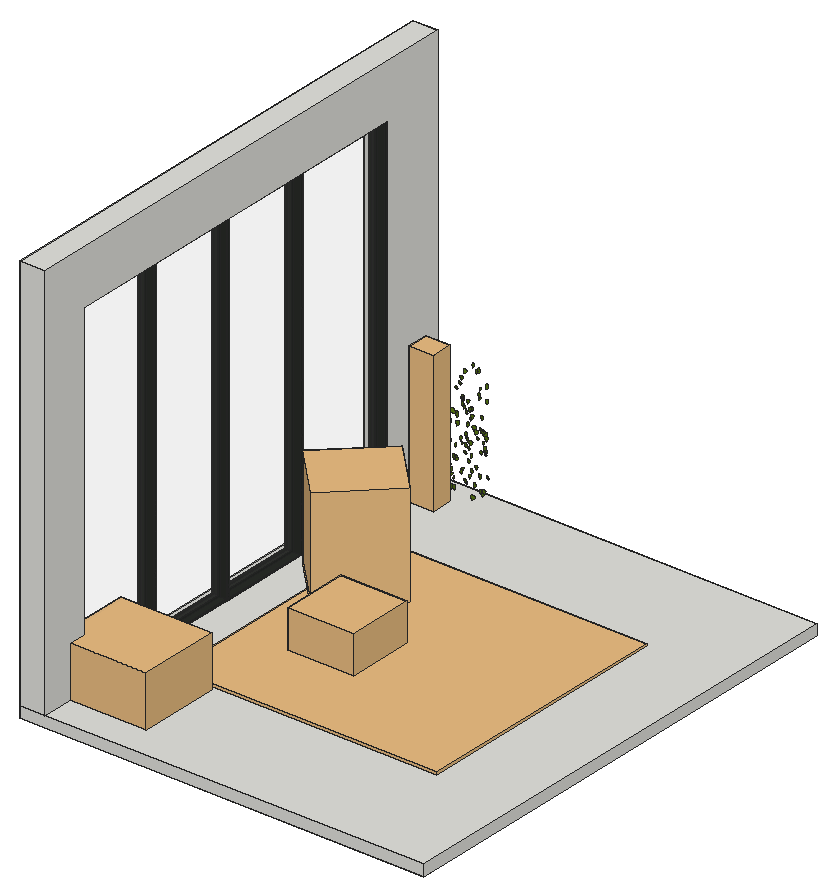
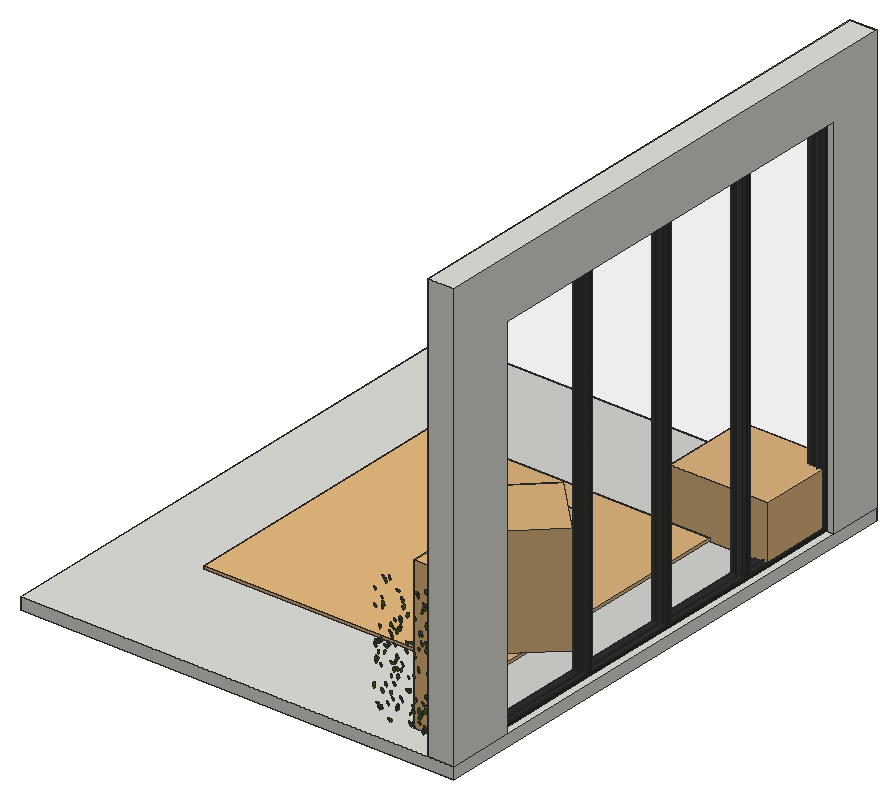
# SketchUp Ruby script. Lengths in inches.
U = 1.inch
M = Sketchup.active_model
def pt(a) = Geom::Point3d.new(a.map { |v| v * U })
def face(e, loops, mat)
  f = e.add_face(loops[0].map { |a| pt(a) })
  loops[1..].each { |l| e.add_face(l.map { |a| pt(a) }).erase! }
  f.material = f.back_material = mat if mat
  f
end
# faces: each face lists its corners as indices into pts; further lists are holes
def faces(e, pts, list, mat = nil) = list.each { |f| face(e, (f[0].is_a?(Array) ? f : [f]).map { |l| l.map { |i| pts[i] } }, mat) }
# xy, xz, yz: faces in a plane at the given z, y or x. An outline is a flat list of corners, or four numbers for a rectangle; further outlines are holes
def ring(l) = l.size == 4 ? [[l[0], l[1]], [l[2], l[1]], [l[2], l[3]], [l[0], l[3]]] : l.each_slice(2).to_a
def flat(e, list, mat, &to3) = list.each { |f| face(e, (f[0].is_a?(Array) ? f : [f]).map { |l| ring(l).map { |u, v| to3.(u, v) } }, mat) }
def xy(e, z, list, mat = nil) = flat(e, list, mat) { |x, y| [x, y, z] }
def xz(e, y, list, mat = nil) = flat(e, list, mat) { |x, z| [x, y, z] }
def yz(e, x, list, mat = nil) = flat(e, list, mat) { |y, z| [x, y, z] }
def lines(e, pts, list) = list.each { |a, b| e.add_line(pt(pts[a]), pt(pts[b])) }
# prism: a flat outline (further loops are holes) pulled along v
def prism(e, loops, v, mat = nil)
  f = face(e, loops, mat); d = Geom::Vector3d.new(v.map { |x| x * U })
  f.pushpull(f.normal.samedirection?(d) ? d.length : -d.length)
end
def box(e, o, s, mat = nil) = prism(e, [[o, [o[0] + s[0], o[1], o[2]], [o[0] + s[0], o[1] + s[1], o[2]], [o[0], o[1] + s[1], o[2]]]], [0, 0, s[2]], mat)
def at(x, y, z, deg = 0) = Geom::Transformation.translation(pt([x, y, z])) * Geom::Transformation.rotation(ORIGIN, Z_AXIS, deg.degrees)
def axes(o, x, y, z) = Geom::Transformation.new([*x, 0, *y, 0, *z, 0, *pt(o).to_a, 1])
def part(name) = M.definitions.add(name)
# library, detail: a bought-in or finely detailed component or shape, given as its bounding box
def library(name, o, s) = part(name).tap { |d| box(d.entities, o, s) }
def detail(e, o, s) = box(e.add_group.entities, o, s)
def put(e, d, t, mat = nil) = e.add_instance(d, t).tap { |i| i.material = mat if mat }
def group(e, t, mat = nil) = e.add_group.tap { |g| g.transformation = t; g.material = mat if mat }.entities
root = M.entities
M.materials.add("Glazing").color = [128, 128, 128]
M.materials["Glazing"].alpha = 0.05
M.materials.add("Powdercoating").color = [41, 44, 40]
M.materials.add("[Vegetation Blur 03]").color = [83, 114, 18]
M.materials.add("grey velvet texture").color = [200, 200, 193]
c1 = library("Potted plant",[-17.58,-15.45,-0.53],[33.42,30.09,19.21])
c2 = library("07",[-18.99,-18.99,0],[37.98,37.98,14.32])
c3 = part("Group\#15")
xy(c3.entities,0,[[0,-55.94,0.71,45.94]])
xy(c3.entities,0.2,[[0,-55.94,0.47,45.94],[0.47,45.94,0.71,46.42]])
xy(c3.entities,2.36,[[0.47,-55.94,0.71,46.42]])
xz(c3.entities,-55.94,[[0,0,0.71,0,0.71,2.36,0.47,2.36,0.47,0.2,0,0.2]])
xz(c3.entities,45.94,[[0,0,0.71,0.2]])
xz(c3.entities,46.42,[[0.47,0.2,0.71,2.36]])
yz(c3.entities,0,[[-55.94,0,45.94,0.2]])
yz(c3.entities,0.47,[[-55.94,0.2,46.42,2.36]])
yz(c3.entities,0.71,[[-55.94,0,45.94,0,45.94,0.2,46.42,0.2,46.42,2.36,-55.94,2.36]])
c4 = part("Group\#7")
xy(c4.entities,0,[[0,-59.09,0.71,45.94]])
xy(c4.entities,0.2,[[0,-59.09,0.47,45.94],[0.47,45.94,0.71,46.42]])
xy(c4.entities,2.36,[[0.47,-59.09,0.71,46.42]])
xz(c4.entities,-59.09,[[0,0,0.71,0,0.71,2.36,0.47,2.36,0.47,0.2,0,0.2]])
xz(c4.entities,45.94,[[0,0,0.71,0.2]])
xz(c4.entities,46.42,[[0.47,0.2,0.71,2.36]])
yz(c4.entities,0,[[-59.09,0,45.94,0.2]])
yz(c4.entities,0.47,[[-59.09,0.2,46.42,2.36]])
yz(c4.entities,0.71,[[-59.09,0,45.94,0,45.94,0.2,46.42,0.2,46.42,2.36,-59.09,2.36]])
c5 = part("Group\#16")
prism(c5.entities,[[[0.47,-56.18,0.2],[0,-56.18,0.2],[0,-56.18,0],[0.71,-56.18,0],[0.71,-56.18,2.36],[0.47,-56.18,2.36]]],[0,28.68,0])
c6 = part("Group\#10")
box(c6.entities,[-0.73,0,0],[27.99,0.55,102.05])
c7 = part("Group\#18")
xy(c7.entities,0,[[0.47,-56.18,0.47,-55.47,0,-55.47,0,-28.21,1.18,-28.21,1.18,-56.18]])
xy(c7.entities,0.2,[[0.71,-56.18,1.18,-28.21],[0,-55.47,0.47,-28.21],[0.47,-28.21,0.71,-27.74]])
xy(c7.entities,2.36,[[0.47,-56.18,0.71,-27.74]])
xz(c7.entities,-56.18,[[0.47,0,1.18,0,1.18,0.2,0.71,0.2,0.71,2.36,0.47,2.36]])
xz(c7.entities,-55.47,[[0,0,0.47,0.2]])
xz(c7.entities,-28.21,[[0,0,1.18,0.2]])
xz(c7.entities,-27.74,[[0.47,0.2,0.71,2.36]])
yz(c7.entities,0,[[-55.47,0,-28.21,0.2]])
yz(c7.entities,0.47,[[-56.18,0,-55.47,0.2],[-56.18,0.2,-27.74,2.36]])
yz(c7.entities,0.71,[[-56.18,0.2,-27.74,2.36]])
yz(c7.entities,1.18,[[-56.18,0,-28.21,0.2]])
c8 = part("Group\#34")
xy(c8.entities,0,[[-20.45,0,7.76,1.22]])
xy(c8.entities,0.06,[[-20.39,0.06,7.7,1.22]])
xy(c8.entities,0.47,[[-19.98,0,7.28,0.06]])
xy(c8.entities,101.89,[[-19.98,0,7.28,0.06]])
xy(c8.entities,102.3,[[-20.39,0.06,7.7,1.22]])
xy(c8.entities,102.36,[[-20.45,0,7.76,1.22]])
xz(c8.entities,0,[[[-20.45,0,7.76,102.36],[-19.98,0.47,7.28,101.89]]])
xz(c8.entities,0.06,[[[-20.39,0.06,7.7,102.3],[-19.98,0.47,7.28,101.89]]])
xz(c8.entities,1.22,[[[-20.45,0,7.76,102.36],[-20.39,0.06,7.7,102.3]]])
yz(c8.entities,-20.45,[[0,0,1.22,102.36]])
yz(c8.entities,-20.39,[[0.06,0.06,1.22,102.3]])
yz(c8.entities,-19.98,[[0,0.47,0.06,101.89]])
yz(c8.entities,7.28,[[0,0.47,0.06,101.89]])
yz(c8.entities,7.7,[[0.06,0.06,1.22,102.3]])
yz(c8.entities,7.76,[[0,0,1.22,102.36]])
c9 = part("Group\#6")
put(c9.entities,c3,axes([27.97,0,7.875],[1,0,0],[0,0,-1],[0,1,0]),"Powdercoating")
put(c9.entities,c4,axes([0.71,0,6.8],[-1,0,0],[0,0,-0.97687],[0,1,0]),"Powdercoating")
put(c9.entities,c5,axes([-27.5,0,-38.07],[0,0,-1],[-1,0,0],[0,1,0]),"Powdercoating")
put(c9.entities,c6,at(1.12,0.35,-38.39),"Glazing")
put(c9.entities,c7,axes([-27.5,0,63.35],[0,0,1],[-1,0,0],[0,1,0]),"Powdercoating")
put(c9.entities,c8,at(20.6875,1.0625,-38.54),"Powdercoating")
c10 = part("Sliding door panels")
put(c10.entities,c9,at(-1.18,4.5,38.86))
g1 = group(c10.entities,at(84.74,4.5,38.86))
put(g1,c3,axes([-27.97,0,7.875],[-1,0,0],[0,0,-1],[0,1,0]),"Powdercoating")
put(g1,c4,axes([-0.71,0,6.8],[1,0,0],[0,0,-0.97687],[0,1,0]),"Powdercoating")
put(g1,c5,axes([27.5,0,-38.07],[0,0,-1],[1,0,0],[0,1,0]),"Powdercoating")
put(g1,c6,axes([-1.12,0.35,-38.39],[-1,0,0],[0,1,0],[0,0,1]),"Glazing")
put(g1,c7,axes([27.5,0,63.35],[0,0,1],[1,0,0],[0,1,0]),"Powdercoating")
put(g1,c8,axes([-20.6875,1.0625,-38.54],[-1,0,0],[0,1,0],[0,0,1]),"Powdercoating")
g2 = group(c10.entities,at(56.0625,4.5,38.86))
put(g2,c3,axes([-27.97,0,7.875],[-1,0,0],[0,0,-1],[0,1,0]),"Powdercoating")
put(g2,c5,axes([27.5,0,-38.07],[0,0,-1],[1,0,0],[0,1,0]),"Powdercoating")
put(g2,c6,axes([-1.12,0.35,-38.39],[-1,0,0],[0,1,0],[0,0,1]),"Glazing")
put(g2,c7,axes([27.5,0,63.35],[0,0,1],[1,0,0],[0,1,0]),"Powdercoating")
put(g2,c8,axes([-20.6875,1.0625,-38.54],[-1,0,0],[0,1,0],[0,0,1]),"Powdercoating")
g3 = group(g2,at(-0.71,0,6.8),"Powdercoating")
xy(g3,-45.34,[[0.47,0.2,0.71,2.36]])
xy(g3,-44.88,[[0,0,0.71,0.2]])
xy(g3,57.73,[[0,0,0.71,0,0.71,2.36,0.47,2.36,0.47,0.2,0,0.2]])
xz(g3,0,[[0,-44.88,0.71,57.73]])
xz(g3,0.2,[[0.47,-45.34,0.71,-44.88],[0,-44.88,0.47,57.73]])
xz(g3,2.36,[[0.47,-45.34,0.71,57.73]])
yz(g3,0,[[0,-44.88,0.2,57.73]])
yz(g3,0.47,[[0.2,-45.34,2.36,57.73]])
yz(g3,0.71,[[0.2,-45.34,2.36,-45.34,2.36,57.73,0,57.73,0,-44.88,0.2,-44.88]])
put(c10.entities,c9,axes([-33.94,4.5,38.86],[1.14218,0,0],[0,1,0],[0,0,1]))
c11 = part("sliding door")
put(c11.entities,c10,at(0,-4.5,-0.08))
c12 = library("Group\#118",[0,0,0],[96,96,0.875])
c13 = library("skpAC60",[-20.16,-58.37,-29.87],[28.24,25.02,29.47])
c14 = library("Vase with branches",[-3.14,-2.52,0],[5.55,4.85,32.04])
c15 = part("ivy")
xy(c15.entities,0,[[0.782,0,0.786,0,0.787,0.005,0.789,0.009,0.821,0.072,0.875,0.147,1.001,0.272,1.073,0.331,1.137,0.363,1.178,0.379,1.223,0.384,1.272,0.383,1.311,0.374,1.36,0.355,1.399,0.334,1.491,0.285,1.541,0.244,1.583,0.199,1.617,0.15,1.64,0.128,1.662,0.115,1.717,0.105,1.745,0.093,1.784,0.054,1.819,0.057,1.854,0.064,1.882,0.075,1.896,0.074,1.91,0.071,1.937,0.063,1.964,0.053,1.99,0.038,2.016,0.015,2.034,0.002,2.04,0,2.038,0.003,2.036,0.007,2.033,0.038,2.036,0.068,2.045,0.1,2.055,0.116,2.064,0.123,2.077,0.129,2.088,0.129,2.106,0.132,2.118,0.13,2.179,0.132,2.207,0.133,2.225,0.133,2.242,0.138,2.22,0.162,2.207,0.186,2.206,0.213,2.212,0.236,2.228,0.262,2.247,0.274,2.298,0.283,2.355,0.294,2.37,0.296,2.376,0.295,2.377,0.3,2.377,0.303,2.385,0.329,2.411,0.37,2.426,0.392,2.449,0.407,2.511,0.426,2.561,0.444,2.619,0.466,2.589,0.469,2.561,0.476,2.501,0.5,2.449,0.516,2.424,0.523,2.401,0.535,2.377,0.556,2.372,0.568,2.36,0.575,2.268,0.586,2.225,0.592,2.207,0.599,2.194,0.61,2.143,0.65,2.13,0.664,2.122,0.682,2.123,0.7,2.13,0.719,2.148,0.75,2.17,0.781,2.195,0.807,2.221,0.828,2.284,0.874,2.291,0.88,2.288,0.887,2.276,0.9,2.267,0.916,2.265,0.933,2.273,0.967,2.292,1.002,2.313,1.03,2.334,1.054,2.348,1.067,2.358,1.074,2.363,1.076,2.362,1.081,2.35,1.094,2.347,1.11,2.35,1.143,2.359,1.18,2.385,1.254,2.415,1.324,2.448,1.393,2.45,1.4,2.446,1.398,2.44,1.394,2.427,1.383,2.402,1.36,2.376,1.339,2.345,1.324,2.305,1.309,2.282,1.303,2.273,1.306,2.245,1.294,2.212,1.287,2.187,1.291,2.163,1.301,2.142,1.316,2.134,1.327,2.124,1.325,2.09,1.292,2.053,1.259,2.014,1.234,1.973,1.215,1.954,1.21,1.931,1.208,1.909,1.212,1.893,1.22,1.879,1.233,1.872,1.248,1.867,1.281,1.864,1.319,1.821,1.258,1.773,1.197,1.726,1.141,1.698,1.121,1.679,1.116,1.666,1.117,1.647,1.122,1.632,1.129,1.62,1.141,1.617,1.154,1.617,1.219,1.621,1.254,1.623,1.268,1.623,1.281,1.618,1.314,1.606,1.346,1.603,1.375,1.607,1.403,1.603,1.467,1.599,1.499,1.605,1.525,1.614,1.552,1.629,1.577,1.635,1.589,1.629,1.587,1.618,1.582,1.596,1.566,1.581,1.556,1.568,1.552,1.557,1.55,1.545,1.553,1.531,1.562,1.522,1.572,1.504,1.591,1.486,1.611,1.474,1.631,1.457,1.666,1.455,1.684,1.457,1.698,1.452,1.715,1.444,1.728,1.424,1.754,1.419,1.772,1.423,1.786,1.434,1.819,1.444,1.848,1.446,1.855,1.44,1.861,1.43,1.867,1.386,1.904,1.349,1.948,1.326,1.973,1.31,1.995,1.288,2.048,1.284,2.153,1.287,2.254,1.284,2.255,1.282,2.253,1.278,2.247,1.274,2.237,1.266,2.216,1.226,2.125,1.208,2.076,1.184,2.033,1.155,1.984,1.135,1.942,1.111,1.899,1.083,1.861,1.053,1.85,1.059,1.83,1.061,1.809,1.056,1.79,1.049,1.767,1.04,1.749,1.018,1.733,0.994,1.726,0.942,1.734,0.95,1.6875,0.944,1.645,0.932,1.608,0.911,1.585,0.881,1.58,0.854,1.582,0.828,1.588,0.785,1.618,0.773,1.625,0.775,1.614,0.779,1.598,0.796,1.502,0.818,1.402,0.861,1.283,0.882,1.224,0.894,1.174,0.892,1.148,0.886,1.123,0.881,1.107,0.872,1.099,0.849,1.094,0.818,1.092,0.789,1.098,0.762,1.107,0.753,1.113,0.721,1.139,0.698,1.163,0.678,1.194,0.665,1.224,0.628,1.28,0.612,1.312,0.606,1.327,0.606,1.314,0.599,1.282,0.594,1.267,0.581,1.256,0.544,1.245,0.512,1.244,0.473,1.249,0.444,1.256,0.382,1.288,0.339,1.306,0.324,1.316,0.317,1.324,0.309,1.326,0.27,1.314,0.227,1.313,0.185,1.3125,0.152,1.317,0.122,1.328,0.092,1.345,0.073,1.353,0.079,1.338,0.092,1.308,0.117,1.249,0.13,1.215,0.139,1.164,0.147,1.148,0.157,1.136,0.163,1.122,0.174,1.086,0.177,1.067,0.182,1.054,0.186,1.043,0.191,1.038,0.211,1.028,0.237,1.005,0.25,0.974,0.253,0.96,0.25,0.944,0.242,0.914,0.243,0.906,0.249,0.902,0.26,0.894,0.289,0.88,0.307,0.873,0.322,0.862,0.364,0.799,0.403,0.738,0.431,0.709,0.439,0.691,0.441,0.678,0.4375,0.66,0.428,0.645,0.394,0.623,0.303,0.594,0.255,0.581,0.214,0.577,0.179,0.573,0.173,0.568,0.175,0.561,0.167,0.55,0.141,0.523,0.113,0.503,0.077,0.49,0.045,0.486,0.026,0.485,0.019,0.486,0.011,0.483,0,0.471,0.014,0.467,0.044,0.455,0.058,0.447,0.07,0.438,0.097,0.411,0.125,0.394,0.158,0.377,0.174,0.366,0.182,0.359,0.185,0.361,0.242,0.331,0.253,0.316,0.258,0.303,0.262,0.283,0.274,0.278,0.308,0.274,0.341,0.252,0.366,0.226,0.366,0.222,0.37,0.22,0.38,0.221,0.395,0.221,0.425,0.216,0.45,0.207,0.465,0.192,0.473,0.178,0.484,0.15,0.489,0.116,0.483,0.089,0.468,0.058,0.45,0.035,0.435,0.018,0.429,0.011,0.434,0.012,0.438,0.014,0.469,0.019,0.542,0.016,0.581,0.015,0.612,0.027,0.68,0.055,0.696,0.057,0.712,0.052,0.73,0.045,0.741,0.036,0.766,0.014]])
xz(root,84.39,[[70.22,5,70.22,5.05,70.21,5.03]])
p = [[70.2,84.4,5],[70.21,84.39,5.03],[71.12,84.21,5],[71.13,84.21,5.03],[71.14,84.21,5],[72.97,83.84,5],
  [72.98,83.84,5.03],[72.05,84.02,5.03],[72.0625,84.02,5],[72.04,84.02,5],[72.98,83.84,5],[73.89,83.65,5],
  [73.9,83.65,5.03],[73.91,83.65,5]]
lines(root,p,[[0,1],[2,3],[3,4],[5,6],[7,8],[9,7],[6,10],[11,12],[12,13]])
put(root,c1,at(21.04,27.2,4))
put(root,c2,axes([52.9375,83.75,5.33],[0.64,0,0],[0,0.64,0],[0,0,0.96]))
put(root,c11,axes([2.57,117.61,4],[0,-1.17539,0],[2.32,0,0],[0,0,1.21966]))
g4 = group(root,at(0,0,4))
prism(g4,[[[9,0,0],[9,18,0],[9,18,126],[9,157.5,126],[9,157.5,0],[9,180,0],[9,180,146],[9,0,146]]],[-9,0,0])
g5 = group(root,at(0,0,0))
box(g5,[0,0,0],[148,180,4])
put(root,c12,at(22.83,42.41,4.5),"grey velvet texture")
put(root,c13,axes([4.71,151.19,43.45],[0.72055,0.6934,0],[-0.6934,0.72055,0],[0,0,1.27]))
put(root,c14,axes([17.72,166.45,4],[1.6,0,0],[0,1.6,0],[0,0,1.6]))
put(root,c15,axes([12.91,173.7,31.39],[0.62306,-0.44776,0.08452],[0.0504,-0.33563,-0.52711],[-0.23565,-1.25564,0.11075]),"[Vegetation Blur 03]")
put(root,c15,axes([22.79,173.7,37.12],[0.43009,-0.41994,0.38446],[0.46829,-0.19735,-0.38284],[-0.21039,-1.29771,-0.06619]),"[Vegetation Blur 03]")
put(root,c15,axes([29.04,173.7,49],[0.61554,-0.40401,-0.01131],[-0.04771,-0.21545,-0.519],[-0.19095,-1.24853,0.09322]),"[Vegetation Blur 03]")
put(root,c15,axes([24.54,173.7,9.62],[0.09448,-0.24372,0.47773],[0.55916,-0.39227,-0.10514],[-0.20978,-1.15536,-0.06508]),"[Vegetation Blur 03]")
put(root,c15,axes([16.85,173.7,24.18],[0.48124,-0.36893,0.30519],[0.35516,-0.24188,-0.41903],[-0.21409,-1.23057,-0.00913]),"[Vegetation Blur 03]")
put(root,c15,axes([22.3125,173.7,24.21],[0.50493,-0.24622,0.19162],[0.19585,-0.34808,-0.41408],[-0.17632,-1.09173,0.08881]),"[Vegetation Blur 03]")
put(root,c15,axes([27.6875,173.7,11.01],[0.55698,-0.45746,-0.14027],[-0.2006,-0.09744,-0.48055],[-0.19678,-1.19551,0.09284]),"[Vegetation Blur 03]")
put(root,c15,axes([20.92,173.7,28.85],[0.61028,-0.27277,0.17175],[0.18054,-0.30337,-0.50308],[-0.17106,-1.2933,0.08178]),"[Vegetation Blur 03]")
put(root,c15,axes([31.43,173.7,21.76],[0.23423,-0.31556,0.37462],[0.44905,-0.24958,-0.22008],[-0.18046,-1.03065,-0.06141]),"[Vegetation Blur 03]")
put(root,c15,axes([24.39,173.7,24.64],[0.40386,-0.35784,0.38449],[0.46593,-0.19708,-0.35483],[-0.18733,-1.26162,-0.05362]),"[Vegetation Blur 03]")
put(root,c15,axes([15.78,173.7,32.88],[0.58162,-0.37165,0.13863],[0.15197,-0.16988,-0.49633],[-0.1959,-1.23523,0.02655]),"[Vegetation Blur 03]")
put(root,c15,axes([23.18,173.7,37.63],[0.38011,-0.35457,0.334],[0.40396,-0.18413,-0.33696],[-0.18436,-1.13452,-0.04969]),"[Vegetation Blur 03]")
put(root,c15,axes([24.25,173.7,33.17],[0.29678,-0.27186,0.42657],[0.50911,-0.26247,-0.26224],[-0.17731,-1.20867,-0.039]),"[Vegetation Blur 03]")
put(root,c15,axes([32.2,173.7,44.81],[0.4979,-0.40473,-0.18477],[-0.2554,-0.09899,-0.42431],[-0.15719,-1.12116,0.10416]),"[Vegetation Blur 03]")
put(root,c15,axes([18.55,173.7,6.63],[0.29467,-0.10714,0.44848],[0.50944,-0.44068,-0.23951],[-0.21249,-1.20507,0.04772]),"[Vegetation Blur 03]")
put(root,c15,axes([14.11,173.7,38.14],[0.18149,-0.29755,0.51892],[0.63719,-0.20751,-0.16715],[-0.13848,-1.34475,-0.08903]),"[Vegetation Blur 03]")
put(root,c15,axes([23.68,173.7,10.5],[0.44878,-0.3413,0.36007],[0.4395,-0.14984,-0.38721],[-0.17027,-1.28634,-0.05043]),"[Vegetation Blur 03]")
put(root,c15,axes([16.5,173.7,35.1875],[0.25712,-0.18798,0.42224],[0.4923,-0.32764,-0.22263],[-0.18343,-1.14283,-0.00563]),"[Vegetation Blur 03]")
put(root,c15,axes([23.98,173.7,25.87],[0.47957,-0.26061,0.31785],[0.37221,-0.23733,-0.40467],[-0.1708,-1.24893,0.01057]),"[Vegetation Blur 03]")
put(root,c15,axes([29.4375,173.7,29.38],[0.56286,-0.41503,0.17137],[0.21267,-0.05627,-0.48669],[-0.19885,-1.23496,-0.03542]),"[Vegetation Blur 03]")
put(root,c15,axes([10.58,173.7,48.42],[0.47356,-0.40672,0.26845],[0.33871,-0.06229,-0.41283],[-0.18036,-1.18486,-0.07045]),"[Vegetation Blur 03]")
put(root,c15,axes([31.29,173.7,22.9],[0.57824,-0.2854,0.09144],[0.09076,-0.20234,-0.48162],[-0.15346,-1.19504,0.05971]),"[Vegetation Blur 03]")
put(root,c15,axes([14.74,173.7,7.04],[0.3696,-0.27711,0.38105],[0.45779,-0.2062,-0.31935],[-0.16294,-1.2079,-0.0329]),"[Vegetation Blur 03]")
put(root,c15,axes([30.64,173.7,25.04],[0.31064,-0.27454,0.24989],[0.28954,-0.20759,-0.27561],[-0.1665,-0.87322,-0.01304]),"[Vegetation Blur 03]")
put(root,c15,axes([16.45,173.7,11.98],[0.55958,-0.3731,0.26041],[0.3198,-0.09162,-0.47837],[-0.18004,-1.32239,-0.04033]),"[Vegetation Blur 03]")
put(root,c15,axes([15.67,173.7,15.21],[0.5074,-0.4678,-0.2898],[-0.37384,0.02954,-0.44347],[-0.19497,-1.27408,0.09613]),"[Vegetation Blur 03]")
put(root,c15,axes([14.65,173.7,45.25],[0.5878,-0.24093,0.03931],[0.02588,-0.23212,-0.48155],[-0.12393,-1.19122,0.08588]),"[Vegetation Blur 03]")
put(root,c15,axes([28.71,173.7,40.22],[0.41734,-0.25524,0.42347],[0.50918,-0.21404,-0.35453],[-0.15923,-1.35344,-0.02379]),"[Vegetation Blur 03]")
put(root,c15,axes([31.48,173.7,26.98],[0.53293,-0.19106,0.2627],[0.2994,-0.28671,-0.43737],[-0.15029,-1.24869,0.06023]),"[Vegetation Blur 03]")
put(root,c15,axes([12.21,173.7,44.97],[0.11866,-0.26117,0.39663],[0.48542,-0.20436,-0.1179],[-0.12904,-1.00894,-0.07879]),"[Vegetation Blur 03]")
put(root,c15,axes([10.93,173.7,25.76],[0.52711,-0.21147,0.33505],[0.39283,-0.25745,-0.4372],[-0.15742,-1.35053,0.03088]),"[Vegetation Blur 03]")
put(root,c15,axes([27.875,173.7,28.24],[0.61381,-0.2023,0.00115],[-0.01893,-0.26118,-0.49641],[-0.09648,-1.23581,0.10472]),"[Vegetation Blur 03]")
put(root,c15,axes([18.1,173.7,27.84],[0.18528,-0.05644,0.53215],[0.61865,-0.42892,-0.15063],[-0.2078,-1.32731,0.02605]),"[Vegetation Blur 03]")
put(root,c15,axes([13.1,173.7,48.48],[0.53111,-0.22481,0.11811],[0.12292,-0.23121,-0.43739],[-0.1333,-1.10892,0.06725]),"[Vegetation Blur 03]")
put(root,c15,axes([31.97,173.7,14.26],[0.31828,-0.32105,0.3684],[0.45752,-0.11523,-0.27908],[-0.137,-1.13071,-0.07616]),"[Vegetation Blur 03]")
put(root,c15,axes([14.1,173.7,33.41],[0.62179,-0.3866,0.07255],[0.08725,-0.03824,-0.53009],[-0.18864,-1.29198,-0.00602]),"[Vegetation Blur 03]")
put(root,c15,axes([26.22,173.7,32.55],[0.51632,-0.17161,0.26126],[0.29868,-0.283,-0.42241],[-0.14219,-1.21766,0.06135]),"[Vegetation Blur 03]")
put(root,c15,axes([15.45,173.7,11.69],[0.16819,-0.22664,0.32974],[0.39401,-0.21788,-0.15742],[-0.14187,-0.87383,-0.04627]),"[Vegetation Blur 03]")
put(root,c15,axes([30.62,173.7,9.62],[0.59208,-0.24793,0.06374],[0.06017,-0.19072,-0.48897],[-0.13036,-1.21404,0.0638]),"[Vegetation Blur 03]")
put(root,c15,axes([17.68,173.7,15.18],[0.5531,-0.30937,0.07702],[0.082,-0.11827,-0.46698],[-0.15743,-1.14854,0.02734]),"[Vegetation Blur 03]")
put(root,c15,axes([23.28,173.7,36.16],[0.42016,-0.3703,-0.17602],[-0.23818,-0.04638,-0.36333],[-0.14889,-0.97076,0.0845]),"[Vegetation Blur 03]")
put(root,c15,axes([22.35,173.7,12.75],[0.26152,-0.04302,0.44662],[0.5117,-0.42542,-0.20602],[-0.19512,-1.17335,0.05832]),"[Vegetation Blur 03]")
put(root,c15,axes([18.02,173.7,14.93],[0.62192,-0.51222,0.08279],[0.13225,0.12501,-0.54004],[-0.23401,-1.29066,-0.08517]),"[Vegetation Blur 03]")
put(root,c15,axes([13.62,173.7,14.91],[0.58633,-0.27865,-0.1062],[-0.1477,-0.14213,-0.48453],[-0.11598,-1.22771,0.08019]),"[Vegetation Blur 03]")
put(root,c15,axes([11.25,173.7,35.28],[0.64635,-0.1795,-0.0483],[-0.07498,-0.25102,-0.52154],[-0.0741,-1.31182,0.10641]),"[Vegetation Blur 03]")
put(root,c15,axes([24.82,173.7,36.9],[0.46976,-0.15316,0.21327],[0.23871,-0.28032,-0.3819],[-0.12977,-1.07007,0.06952]),"[Vegetation Blur 03]")
put(root,c15,axes([15.77,173.7,35.25],[0.21062,-0.15839,0.41958],[0.49728,-0.27124,-0.18238],[-0.15148,-1.11064,-0.0153]),"[Vegetation Blur 03]")
put(root,c15,axes([27.76,173.7,16.1],[0.40591,-0.18014,0.3374],[0.39655,-0.24525,-0.33836],[-0.14603,-1.16675,0.01903]),"[Vegetation Blur 03]")
put(root,c15,axes([20.1,173.7,17.2],[0.43914,-0.29657,0.03896],[0.03337,-0.10478,-0.37595],[-0.14811,-0.90294,0.03083]),"[Vegetation Blur 03]")
put(root,c15,axes([25.11,173.7,21.45],[0.34584,-0.27967,0.31588],[0.38688,-0.124,-0.2994],[-0.13639,-1.06088,-0.04828]),"[Vegetation Blur 03]")
put(root,c15,axes([28.99,173.7,14.03],[0.57796,-0.29472,0.19025],[0.2281,-0.10009,-0.48593],[-0.15109,-1.27852,-0.00582]),"[Vegetation Blur 03]")
put(root,c15,axes([12.25,173.7,35.73],[0.12614,-0.2409,0.28031],[0.3435,-0.16191,-0.12485],[-0.11696,-0.73532,-0.06434]),"[Vegetation Blur 03]")
put(root,c15,axes([21.94,173.7,41.39],[0.07798,-0.22712,0.49701],[0.61066,-0.17712,-0.07655],[-0.10063,-1.25091,-0.0794]),"[Vegetation Blur 03]")
put(root,c15,axes([27.875,173.7,47.55],[0.32606,-0.15993,0.37004],[0.43652,-0.25327,-0.27342],[-0.14515,-1.12098,0.00898]),"[Vegetation Blur 03]")
put(root,c15,axes([22.22,173.7,44.07],[0.58958,-0.29849,0.19052],[0.22934,-0.09222,-0.49546],[-0.15145,-1.30163,-0.00859]),"[Vegetation Blur 03]")
put(root,c15,axes([18.62,173.7,12.37],[0.33688,-0.08622,0.33874],[0.38873,-0.33347,-0.27086],[-0.15137,-1.04826,0.0583]),"[Vegetation Blur 03]")
put(root,c15,axes([26.79,173.7,29.15],[0.58365,-0.1286,0.23072],[0.26562,-0.28309,-0.47237],[-0.11521,-1.30414,0.07979]),"[Vegetation Blur 03]")
put(root,c15,axes([25.01,173.7,17.51],[0.49387,-0.24848,0.14861],[0.17062,-0.13992,-0.41447],[-0.13648,-1.07408,0.01961]),"[Vegetation Blur 03]")
put(root,c15,axes([32.1875,173.7,39.75],[0.44457,-0.30415,-0.24459],[-0.31847,-0.07486,-0.37092],[-0.10118,-1.10076,0.09281]),"[Vegetation Blur 03]")
put(root,c15,axes([17.73,173.7,48.4],[0.54958,-0.28156,-0.28314],[-0.3622,-0.10008,-0.45262],[-0.08884,-1.33367,0.09374]),"[Vegetation Blur 03]")
put(root,c15,axes([25.5,173.7,12.68],[0.45593,-0.14871,0.15697],[0.17169,-0.25336,-0.36992],[-0.11285,-0.98625,0.07136]),"[Vegetation Blur 03]")
put(root,c15,axes([30.42,173.7,28.92],[0.52102,-0.20474,0.04178],[0.03433,-0.18504,-0.42777],[-0.1065,-1.06132,0.06652]),"[Vegetation Blur 03]")
put(root,c15,axes([16.59,173.7,8.6],[0.49081,-0.25055,0.00673],[-0.00728,-0.13032,-0.40947],[-0.12182,-1.0017,0.05159]),"[Vegetation Blur 03]")
put(root,c15,axes([11.15,173.7,40.7],[0.32628,-0.20206,0.40603],[0.49033,-0.18475,-0.27691],[-0.12932,-1.21026,-0.02552]),"[Vegetation Blur 03]")
put(root,c15,axes([14.52,173.7,16.98],[0.30081,-0.15518,0.1985],[0.21889,-0.23826,-0.25024],[-0.13012,-0.75955,0.03794]),"[Vegetation Blur 03]")
put(root,c15,axes([12.36,173.7,6.41],[0.52824,-0.2088,0.07813],[0.0803,-0.17577,-0.43551],[-0.11407,-1.09065,0.05523]),"[Vegetation Blur 03]")
put(root,c15,axes([23.66,173.7,19.6875],[0.38346,-0.30784,0.36497],[0.45646,-0.05536,-0.32679],[-0.11835,-1.21097,-0.07784]),"[Vegetation Blur 03]")
put(root,c15,axes([30.97,173.7,28.58],[0.64177,-0.16774,0.0763],[0.07979,-0.21804,-0.52237],[-0.09498,-1.31665,0.07678]),"[Vegetation Blur 03]")
put(root,c15,axes([20.83,173.7,17.54],[0.50163,-0.24569,-0.26541],[-0.34021,-0.12729,-0.40976],[-0.06534,-1.2236,0.09592]),"[Vegetation Blur 03]")
put(root,c15,axes([10.78,173.7,11.27],[0.44114,-0.2833,-0.10477],[-0.14493,-0.08165,-0.37173],[-0.12012,-0.94191,0.06374]),"[Vegetation Blur 03]")
put(root,c15,axes([15.35,173.7,6.19],[0.53858,-0.252,0.05397],[0.05479,-0.1161,-0.44944],[-0.12794,-1.11057,0.03474]),"[Vegetation Blur 03]")
put(root,c15,axes([25.27,173.7,29.92],[0.4464,-0.35085,-0.18371],[-0.23796,-0.0009,-0.38487],[-0.15203,-1.02878,0.06299]),"[Vegetation Blur 03]")
put(root,c15,axes([19.64,173.7,16.97],[0.15407,-0.1087,0.33806],[0.39127,-0.27976,-0.13293],[-0.14585,-0.86534,0.00051]),"[Vegetation Blur 03]")
put(root,c15,axes([23.96,173.7,46.85],[0.51677,-0.16,-0.11108],[-0.14975,-0.2188,-0.41446],[-0.04632,-1.0777,0.10064]),"[Vegetation Blur 03]")
put(root,c15,axes([25.38,173.7,34.13],[0.31073,-0.06738,0.37222],[0.4328,-0.32267,-0.24985],[-0.14749,-1.08882,0.05101]),"[Vegetation Blur 03]")
put(root,c15,axes([16.02,173.7,11.26],[0.4884,-0.38994,-0.09349],[-0.11293,0.05241,-0.42733],[-0.19047,-1.03097,0.01363]),"[Vegetation Blur 03]")
put(root,c15,axes([19.625,173.7,32.56],[0.49181,-0.15671,-0.3315],[-0.41314,-0.21702,-0.39213],[0.00973,-1.29451,0.10587]),"[Vegetation Blur 03]")
put(root,c15,axes([16.625,173.7,31.01],[0.44605,-0.17185,0.11357],[0.12178,-0.19918,-0.36599],[-0.10728,-0.94065,0.05675]),"[Vegetation Blur 03]")
put(root,c15,axes([30.53,173.7,8.57],[0.42261,-0.28747,-0.1193],[-0.16204,-0.06467,-0.35783],[-0.12093,-0.91792,0.06257]),"[Vegetation Blur 03]")
put(root,c15,axes([14.2,173.7,30.62],[0.10022,-0.2222,0.4688],[0.57871,-0.13035,-0.09212],[-0.08191,-1.19279,-0.07727]),"[Vegetation Blur 03]")
put(root,c15,axes([18.48,173.7,21.9],[0.3651,-0.20886,0.13721],[0.15459,-0.14475,-0.30864],[-0.12111,-0.81437,0.01967]),"[Vegetation Blur 03]")
put(root,c15,axes([22.65,173.7,37.11],[0.28904,-0.06987,0.39444],[0.46239,-0.30604,-0.23421],[-0.14468,-1.11768,0.03947]),"[Vegetation Blur 03]")
put(root,c15,axes([26.36,173.7,6.21],[0.65317,-0.15035,0.08957],[0.09783,-0.2124,-0.5313],[-0.08838,-1.34629,0.07382]),"[Vegetation Blur 03]")
put(root,c15,axes([19.35,173.7,6.98],[0.51611,-0.14167,0.29822],[0.35265,-0.22138,-0.42305],[-0.1179,-1.28232,0.04009]),"[Vegetation Blur 03]")
put(root,c15,axes([13.69,173.7,23.81],[0.1731,-0.14266,0.38005],[0.45428,-0.21748,-0.15066],[-0.12362,-0.99891,-0.02148]),"[Vegetation Blur 03]")
put(root,c15,axes([29.4,173.7,8.52],[0.23742,-0.1267,0.33587],[0.39552,-0.23419,-0.20013],[-0.12927,-0.94922,0.00454]),"[Vegetation Blur 03]")
put(root,c15,axes([20.47,173.7,39.72],[0.30187,-0.29092,0.34167],[0.43037,-0.04293,-0.25902],[-0.10016,-1.06123,-0.08319]),"[Vegetation Blur 03]")
put(root,c15,axes([30.86,173.7,23.55],[0.46252,-0.08041,0.20679],[0.23593,-0.28736,-0.36906],[-0.10033,-1.0465,0.08545]),"[Vegetation Blur 03]")
put(root,c15,axes([18.02,173.7,39.49],[0.34266,-0.16677,0.2483],[0.29126,-0.18349,-0.28712],[-0.11956,-0.92493,0.01219]),"[Vegetation Blur 03]")
put(root,c15,axes([29.3,173.7,39.36],[0.35292,-0.17211,0.08002],[0.07901,-0.17569,-0.29156],[-0.10181,-0.73298,0.0511]),"[Vegetation Blur 03]")
put(root,c15,axes([18.59,173.7,11.41],[0.56213,-0.17838,-0.00831],[-0.02255,-0.16495,-0.45927],[-0.08432,-1.14512,0.06745]),"[Vegetation Blur 03]")
put(root,c15,axes([14.16,173.7,16.9],[0.37075,-0.20222,0.27738],[0.33431,-0.13128,-0.31269],[-0.11578,-1.02663,-0.01465]),"[Vegetation Blur 03]")
put(root,c15,axes([20.23,173.7,20.86],[0.29156,-0.09126,0.22735],[0.25627,-0.25873,-0.23525],[-0.11785,-0.78843,0.05088]),"[Vegetation Blur 03]")
put(root,c15,axes([16.43,173.7,9.65],[0.28606,-0.20547,0.36321],[0.44363,-0.1257,-0.24391],[-0.10592,-1.08138,-0.04066]),"[Vegetation Blur 03]")
put(root,c15,axes([30.21,173.7,28.59],[0.31137,-0.19726,0.4006],[0.48849,-0.13513,-0.26337],[-0.10722,-1.1885,-0.03655]),"[Vegetation Blur 03]")
put(root,c15,axes([14.71,173.7,44.08],[0.56579,-0.26175,0.06944],[0.08066,-0.05979,-0.47321],[-0.13005,-1.17586,0.0086]),"[Vegetation Blur 03]")
put(root,c15,axes([26.08,173.7,34.95],[0.39018,-0.19806,0.28181],[0.33951,-0.13277,-0.32778],[-0.115,-1.06391,-0.01155]),"[Vegetation Blur 03]")
put(root,c15,axes([29.98,173.7,33.7],[0.59158,-0.31026,-0.0564],[-0.07139,-0.00087,-0.49803],[-0.1497,-1.22563,0.01463]),"[Vegetation Blur 03]")
put(root,c15,axes([14.4,173.7,6.4],[0.19741,-0.09695,0.50499],[0.60705,-0.24693,-0.16553],[-0.12869,-1.3135,-0.00615]),"[Vegetation Blur 03]")
put(root,c15,axes([12.92,173.7,27.2],[0.23432,-0.21265,0.28086],[0.3439,-0.11223,-0.20448],[-0.10411,-0.84934,-0.0433]),"[Vegetation Blur 03]")
put(root,c15,axes([25.81,173.7,23.98],[0.58607,-0.17658,0.01299],[0.00501,-0.15402,-0.47969],[-0.08713,-1.19658,0.05983]),"[Vegetation Blur 03]")
put(root,c15,axes([29.42,173.7,42.2],[0.24496,-0.07431,0.21292],[0.23492,-0.26987,-0.19483],[-0.11909,-0.6852,0.05364]),"[Vegetation Blur 03]")
put(root,c15,axes([24.98,173.7,23.75],[0.21308,-0.12887,0.25392],[0.29486,-0.2048,-0.18116],[-0.11737,-0.74847,0.00585]),"[Vegetation Blur 03]")
put(root,c15,axes([14.53,173.7,12.14],[0.09309,-0.2572,0.47512],[0.59358,-0.05541,-0.08218],[-0.0469,-1.21192,-0.09707]),"[Vegetation Blur 03]")
put(root,c15,axes([26.12,173.7,18.98],[0.16191,-0.03187,0.41572],[0.48687,-0.31523,-0.1301],[-0.15054,-1.05373,0.02635]),"[Vegetation Blur 03]")
put(root,c15,axes([23.35,173.7,34.96],[0.51145,-0.25079,0.06105],[0.06998,-0.0596,-0.42899],[-0.12471,-1.06199,0.00966]),"[Vegetation Blur 03]")
put(root,c15,axes([21.375,173.7,32.05],[0.48032,-0.40321,-0.3461],[-0.42858,0.11763,-0.41773],[-0.18586,-1.31325,0.06885]),"[Vegetation Blur 03]")
put(root,c15,axes([12.32,173.7,45.49],[0.45619,-0.27219,-0.21417],[-0.27378,-0.03129,-0.38217],[-0.10679,-1.08253,0.0649]),"[Vegetation Blur 03]")
put(root,c15,axes([19.89,173.7,10.15],[0.27567,-0.18278,0.07916],[0.08,-0.13493,-0.23455],[-0.1044,-0.58604,0.02931]),"[Vegetation Blur 03]")
put(root,c15,axes([15.7,173.7,42.58],[0.31604,-0.28517,0.16056],[0.20748,-0.01555,-0.27638],[-0.12189,-0.7659,-0.05417]),"[Vegetation Blur 03]")
put(root,c15,axes([25.82,173.7,31.4375],[0.37901,-0.24998,0.16924],[0.20826,-0.05609,-0.32368],[-0.11995,-0.88726,-0.02722]),"[Vegetation Blur 03]")
put(root,c15,axes([26.76,173.7,48.75],[0.0835,-0.00667,0.46395],[0.54474,-0.33722,-0.06606],[-0.16259,-1.13325,0.01693]),"[Vegetation Blur 03]")
put(root,c15,axes([14.16,173.7,48.87],[0.27432,-0.11887,0.39101],[0.46845,-0.2067,-0.22879],[-0.11587,-1.1171,0.00072]),"[Vegetation Blur 03]")
put(root,c15,axes([24.125,173.7,22.82],[0.56324,-0.31646,-0.09717],[-0.11977,0.02711,-0.47626],[-0.15324,-1.18433,0.01506]),"[Vegetation Blur 03]")
put(root,c15,axes([28.62,173.7,25.57],[0.07402,-0.1812,0.31745],[0.39109,-0.12634,-0.07209],[-0.07805,-0.80492,-0.06015]),"[Vegetation Blur 03]")
put(root,c15,axes([22.86,173.7,22.17],[0.15681,-0.19135,0.27864],[0.34217,-0.11382,-0.14055],[-0.09017,-0.7647,-0.0488]),"[Vegetation Blur 03]")
put(root,c15,axes([26.21,173.7,13.8125],[0.12637,-0.06641,0.44261],[0.52763,-0.25805,-0.10643],[-0.12947,-1.11645,-0.00173]),"[Vegetation Blur 03]")
put(root,c15,axes([16.89,173.7,46.66],[0.3032,0.00804,0.42723],[0.50376,-0.343,-0.23711],[-0.14236,-1.19666,0.07083]),"[Vegetation Blur 03]")
put(root,c15,axes([23.07,173.7,13.79],[0.24227,-0.06001,0.24324],[0.27574,-0.26297,-0.19314],[-0.11679,-0.74533,0.04856]),"[Vegetation Blur 03]")
put(root,c15,axes([11.82,173.7,45.6],[0.40522,-0.15446,0.13943],[0.15914,-0.15283,-0.3347],[-0.09744,-0.89194,0.0332]),"[Vegetation Blur 03]")
put(root,c15,axes([29.64,173.7,21.59],[0.33061,-0.13828,0.23143],[0.27228,-0.16795,-0.27487],[-0.10387,-0.88042,0.01609]),"[Vegetation Blur 03]")
